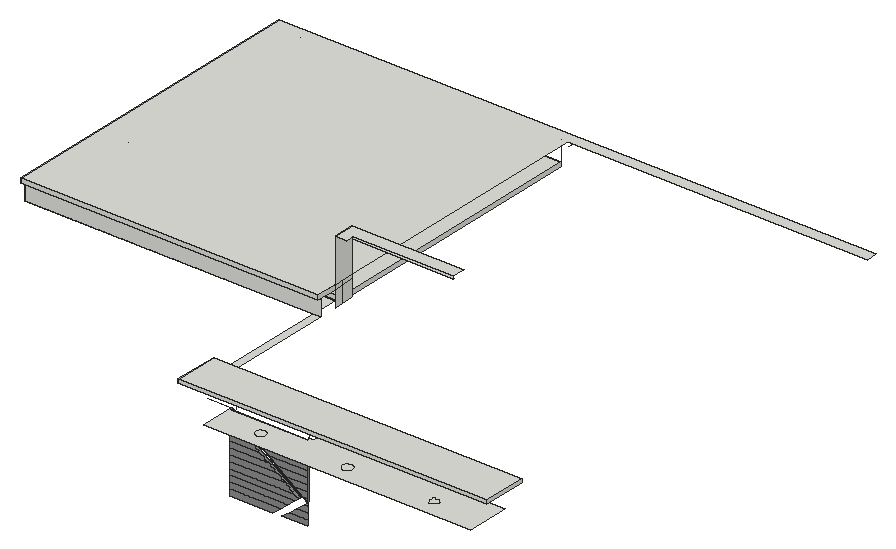
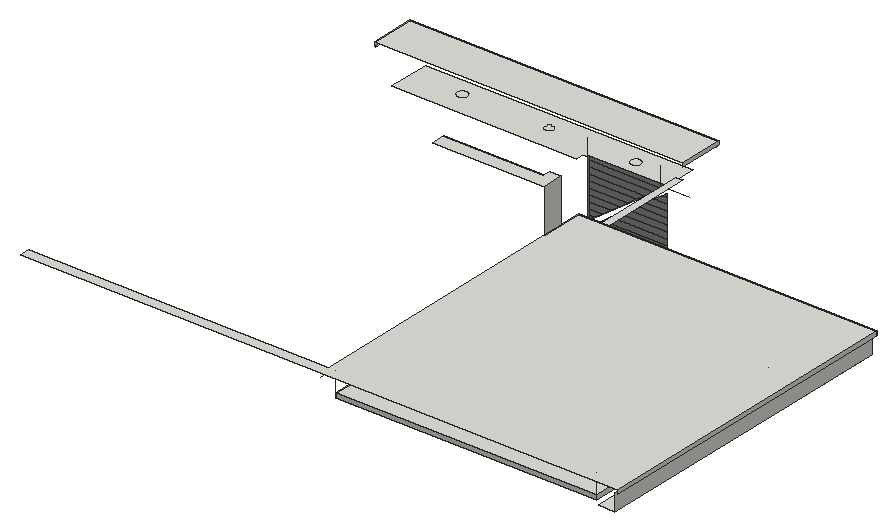
# SketchUp Ruby script. Lengths in inches.
U = 1.inch
M = Sketchup.active_model
def pt(a) = Geom::Point3d.new(a.map { |v| v * U })
def face(e, loops, mat)
  f = e.add_face(loops[0].map { |a| pt(a) })
  loops[1..].each { |l| e.add_face(l.map { |a| pt(a) }).erase! }
  f.material = f.back_material = mat if mat
  f
end
# faces: each face lists its corners as indices into pts; further lists are holes
def faces(e, pts, list, mat = nil) = list.each { |f| face(e, (f[0].is_a?(Array) ? f : [f]).map { |l| l.map { |i| pts[i] } }, mat) }
# xy, xz, yz: faces in a plane at the given z, y or x. An outline is a flat list of corners, or four numbers for a rectangle; further outlines are holes
def ring(l) = l.size == 4 ? [[l[0], l[1]], [l[2], l[1]], [l[2], l[3]], [l[0], l[3]]] : l.each_slice(2).to_a
def flat(e, list, mat, &to3) = list.each { |f| face(e, (f[0].is_a?(Array) ? f : [f]).map { |l| ring(l).map { |u, v| to3.(u, v) } }, mat) }
def xy(e, z, list, mat = nil) = flat(e, list, mat) { |x, y| [x, y, z] }
def xz(e, y, list, mat = nil) = flat(e, list, mat) { |x, z| [x, y, z] }
def yz(e, x, list, mat = nil) = flat(e, list, mat) { |y, z| [x, y, z] }
def lines(e, pts, list) = list.each { |a, b| e.add_line(pt(pts[a]), pt(pts[b])) }
# prism: a flat outline (further loops are holes) pulled along v
def prism(e, loops, v, mat = nil)
  f = face(e, loops, mat); d = Geom::Vector3d.new(v.map { |x| x * U })
  f.pushpull(f.normal.samedirection?(d) ? d.length : -d.length)
end
def box(e, o, s, mat = nil) = prism(e, [[o, [o[0] + s[0], o[1], o[2]], [o[0] + s[0], o[1] + s[1], o[2]], [o[0], o[1] + s[1], o[2]]]], [0, 0, s[2]], mat)
def at(x, y, z, deg = 0) = Geom::Transformation.translation(pt([x, y, z])) * Geom::Transformation.rotation(ORIGIN, Z_AXIS, deg.degrees)
def axes(o, x, y, z) = Geom::Transformation.new([*x, 0, *y, 0, *z, 0, *pt(o).to_a, 1])
def part(name) = M.definitions.add(name)
# library, detail: a bought-in or finely detailed component or shape, given as its bounding box
def library(name, o, s) = part(name).tap { |d| box(d.entities, o, s) }
def detail(e, o, s) = box(e.add_group.entities, o, s)
def put(e, d, t, mat = nil) = e.add_instance(d, t).tap { |i| i.material = mat if mat }
def group(e, t, mat = nil) = e.add_group.tap { |g| g.transformation = t; g.material = mat if mat }.entities
root = M.entities
M.materials.add("[0129_WhiteSmoke]").color = [245, 245, 245]
M.materials.add("[Color M04]").color = [142, 142, 142]
prism(root,[[[207.97,182.25,490.625],[194.85,182.25,490.625],[24.875,182.25,490.625],[24.875,233.22,490.625],[24.875,250.625,490.625],[24.875,411,490.625],[241.25,411,490.625],[241.25,182.25,490.625]]],[0,0,3.375])
xy(root,479,[[[261.37,15.6875,261.37,42.75,325.49,42.75,325.49,44.6875,329.48,44.6875,329.48,50.6875,482.9375,50.6875,482.9375,15.6875],[296.29,26.3,297.34,26.31,298.34,26.58,299.25,27.1,299.98,27.84,300.5,28.75,300.77,29.76,300.77,30.8,300.49,31.8125,299.97,32.71,299.23,33.45,298.32,33.97,297.3125,34.24,296.27,34.23,295.26,33.96,294.36,33.4375,293.62,32.7,293.1,31.79,292.84,30.78,292.84,29.74,293.11,28.73,293.64,27.83,294.38,27.09,295.28,26.57],[368.29,26.3,369.34,26.31,370.34,26.58,371.25,27.1,371.98,27.84,372.5,28.75,372.77,29.76,372.77,30.8,372.49,31.8125,371.97,32.71,371.23,33.45,370.32,33.97,369.3125,34.24,368.27,34.23,367.26,33.96,366.36,33.4375,365.62,32.7,365.1,31.79,364.84,30.78,364.84,29.74,365.11,28.73,365.64,27.83,366.38,27.09,367.28,26.57],[440.29,26.3,441.34,26.31,442.34,26.58,443.25,27.1,443.98,27.84,444.5,28.75,444.77,29.76,444.77,30.8,444.49,31.8125,443.97,32.71,443.23,33.45,442.32,33.97,441.3125,34.24,440.27,34.23,439.26,33.96,438.36,33.4375,437.62,32.7,437.1,31.79,436.84,30.78,436.84,29.74,437.11,28.73,437.64,27.83,438.38,27.09,439.28,26.57],[333.11,46.6875,333.32,46.71,333.52,46.77,333.7,46.88,333.86,47.02,333.98,47.1875,334.0625,47.38,334.11,47.58,334.11,47.79,334.0625,48,333.98,48.1875,333.86,48.36,333.7,48.5,333.52,48.6,333.32,48.67,333.11,48.6875,332.91,48.67,332.71,48.6,332.53,48.5,332.37,48.36,332.25,48.1875,332.16,48,332.12,47.79,332.12,47.58,332.16,47.38,332.25,47.1875,332.37,47.02,332.53,46.88,332.71,46.77,332.91,46.71]],[296.29,26.3,295.28,26.57,294.38,27.09,293.64,27.83,293.11,28.73,292.84,29.74,292.84,30.78,293.1,31.79,293.62,32.7,294.36,33.4375,295.26,33.96,296.27,34.23,297.3125,34.24,298.32,33.97,299.23,33.45,299.97,32.71,300.49,31.8125,300.77,30.8,300.77,29.76,300.5,28.75,299.98,27.84,299.25,27.1,298.34,26.58,297.34,26.31],[368.29,26.3,367.28,26.57,366.38,27.09,365.64,27.83,365.11,28.73,364.84,29.74,364.84,30.78,365.1,31.79,365.62,32.7,366.36,33.4375,367.26,33.96,368.27,34.23,369.3125,34.24,370.32,33.97,371.23,33.45,371.97,32.71,372.49,31.8125,372.77,30.8,372.77,29.76,372.5,28.75,371.98,27.84,371.25,27.1,370.34,26.58,369.34,26.31],[440.29,26.3,439.28,26.57,438.38,27.09,437.64,27.83,437.11,28.73,436.84,29.74,436.84,30.78,437.1,31.79,437.62,32.7,438.36,33.4375,439.26,33.96,440.27,34.23,441.3125,34.24,442.32,33.97,443.23,33.45,443.97,32.71,444.49,31.8125,444.77,30.8,444.77,29.76,444.5,28.75,443.98,27.84,443.25,27.1,442.34,26.58,441.34,26.31]])
xy(root,494,[[241.25,50.6875,247.25,154.25],[[2.0625,154.25,2.0625,420,15.875,420,15.875,176.25,241.25,176.25,241.25,154.25],[121.1,160.82,122.13,160.96,123.1,161.36,123.93,161.99,124.5625,162.82,124.96,163.78,125.1,164.82,124.96,165.85,124.5625,166.82,123.93,167.65,123.1,168.28,122.13,168.68,121.1,168.82,120.0625,168.68,119.1,168.28,118.27,167.65,117.63,166.82,117.23,165.85,117.1,164.82,117.23,163.78,117.63,162.82,118.27,161.99,119.1,161.36,120.0625,160.96],[43.23,160.82,44.27,160.96,45.23,161.36,46.0625,161.99,46.7,162.82,47.1,163.78,47.23,164.82,47.1,165.85,46.7,166.82,46.0625,167.65,45.23,168.28,44.27,168.68,43.23,168.82,42.2,168.68,41.23,168.28,40.4,167.65,39.77,166.82,39.37,165.85,39.23,164.82,39.37,163.78,39.77,162.82,40.4,161.99,41.23,161.36,42.2,160.96]],[43.23,160.82,42.2,160.96,41.23,161.36,40.4,161.99,39.77,162.82,39.37,163.78,39.23,164.82,39.37,165.85,39.77,166.82,40.4,167.65,41.23,168.28,42.2,168.68,43.23,168.82,44.27,168.68,45.23,168.28,46.0625,167.65,46.7,166.82,47.1,165.85,47.23,164.82,47.1,163.78,46.7,162.82,46.0625,161.99,45.23,161.36,44.27,160.96],[121.1,160.82,120.0625,160.96,119.1,161.36,118.27,161.99,117.63,162.82,117.23,163.78,117.1,164.82,117.23,165.85,117.63,166.82,118.27,167.65,119.1,168.28,120.0625,168.68,121.1,168.82,122.13,168.68,123.1,168.28,123.93,167.65,124.5625,166.82,124.96,165.85,125.1,164.82,124.96,163.78,124.5625,162.82,123.93,161.99,123.1,161.36,122.13,160.96]])
xy(root,503.875,[[241.25,13.9375,241.25,15.6875,495.875,15.6875,495.875,50.6875,497.375,50.6875,497.375,13.9375]])
xy(root,506.875,[[241.25,13.9375,497.375,50.6875]])
xy(root,507.4375,[[0,151.75,0,420,2.0625,420,2.0625,154.25,247.25,154.25,247.25,151.75]])
xy(root,511,[[0,151.75,247.25,151.75,247.25,411,495.875,411,495.875,420,0,420]])
xy(root,545.23,[[256.62,175.6875,339.9375,176.25]],"[0129_WhiteSmoke]")
xy(root,547.1875,[[247.25,169.5,256.62,169.5,256.62,175.6875,339.9375,175.6875,339.9375,187,247.25,187]])
xz(root,13.9375,[[241.25,503.875,497.375,506.875]])
xz(root,42.75,[[261.37,414.42,297.02,414.42,303.14,419.54,261.37,419.54],[304.39,414.42,325.49,414.42,325.49,419.54,310.6,419.54],[261.37,419.54,303.14,419.54,309.27,424.67,261.37,424.67],[310.6,419.54,325.49,419.54,325.49,424.67,316.8,424.67],[261.37,424.67,309.27,424.67,315.4,429.79,261.37,429.79],
  [316.8,424.67,325.49,424.67,325.49,429.79,323.01,429.79],[261.37,429.79,315.4,429.79,318.21,432.15,314.39,434.92,261.37,434.92],[323.01,429.79,325.49,429.79,325.49,431.84],[325.49,431.84,325.49,434.92,321.3,434.92],[261.37,434.92,314.39,434.92,307.31,440.04,261.37,440.04],
  [321.3,434.92,325.49,434.92,325.49,440.04,314.33,440.04],[261.37,440.04,307.31,440.04,300.24,445.17,261.37,445.17],[314.33,440.04,325.49,440.04,325.49,445.17,307.37,445.17],[261.37,445.17,300.24,445.17,293.16,450.29,261.37,450.29],[307.37,445.17,325.49,445.17,325.49,450.29,300.4,450.29],
  [261.37,450.29,293.16,450.29,286.09,455.42,261.37,455.42],[300.4,450.29,325.49,450.29,325.49,455.42,293.43,455.42],[261.37,455.42,286.09,455.42,279.01,460.54,261.37,460.54],[293.43,455.42,325.49,455.42,325.49,460.54,286.46,460.54],[261.37,460.54,279.01,460.54,271.9375,465.67,261.37,465.67],
  [286.46,460.54,325.49,460.54,325.49,465.67,279.5,465.67],[261.37,465.67,271.9375,465.67,264.86,470.8,261.37,470.8],[279.5,465.67,325.49,465.67,325.49,470.79,272.53,470.79],[272.53,470.79,325.49,470.79,325.49,475.92,265.5625,475.92],[261.37,470.8,264.86,470.8,261.37,473.32],
  [265.5625,475.92,325.49,475.92,325.49,479,261.37,479]],"[Color M04]")
xz(root,151.75,[[0,507.4375,247.25,511]])
xz(root,154.25,[[2.0625,494,247.25,507.4375]])
xz(root,175.6875,[[256.62,545.23,339.9375,547.1875]],"[0129_WhiteSmoke]")
yz(root,0,[[151.75,507.4375,420,511]])
yz(root,2.0625,[[154.25,494,420,507.4375]])
yz(root,241.25,[[13.9375,503.875,50.6875,506.875]])
yz(root,247.25,[[169.5,494,176.25,507.4375],[176.25,494,187,507.4375],[151.75,507.4375,169.5,511],[169.5,507.4375,176.25,511],[176.25,507.4375,187,511],
  [169.5,511,187,547.1875]])
yz(root,325.49,[[42.75,431.84,44.6875,479]],"[Color M04]")
yz(root,497.375,[[13.9375,503.875,50.6875,506.875]])
p = [[261.37,44.6875,479],[325.49,44.6875,431.84],[325.49,42.75,431.84],[321.3,42.75,434.92],[314.33,42.75,440.04],[307.37,42.75,445.17],
  [300.4,42.75,450.29],[293.43,42.75,455.42],[286.46,42.75,460.54],[279.5,42.75,465.67],[272.53,42.75,470.79],[265.5625,42.75,475.92],
  [261.37,42.75,479],[318.21,44.6875,432.15],[261.37,44.6875,473.32],[261.37,42.75,473.32],[264.86,42.75,470.8],[271.9375,42.75,465.67],
  [279.01,42.75,460.54],[286.09,42.75,455.42],[293.16,42.75,450.29],[300.24,42.75,445.17],[307.31,42.75,440.04],[314.39,42.75,434.92],
  [318.21,42.75,432.15],[265.06,44.6875,494],[265.06,44.6875,479],[325.49,44.6875,494],[325.49,44.6875,479],[24.875,182.25,494],
  [24.875,176.25,494],[247.25,176.25,494],[241.25,176.25,494],[24.875,233.22,494],[24.875,233.22,511],[24.875,411,494],
  [24.875,411,511],[241.25,411,494],[241.25,411,511],[247.25,411,507.4375],[247.25,420,507.4375],[241.25,44.6875,479]]
faces(root,p,[[0,1,2,3,4,5,6,7,8,9,10,11,12],[13,14,15,16,17,18,19,20,21,22,23,24]],"[Color M04]")
lines(root,p,[[25,26],[27,28],[29,30],[31,32],[33,34],[35,36],[37,38],[39,40],[0,41]])
